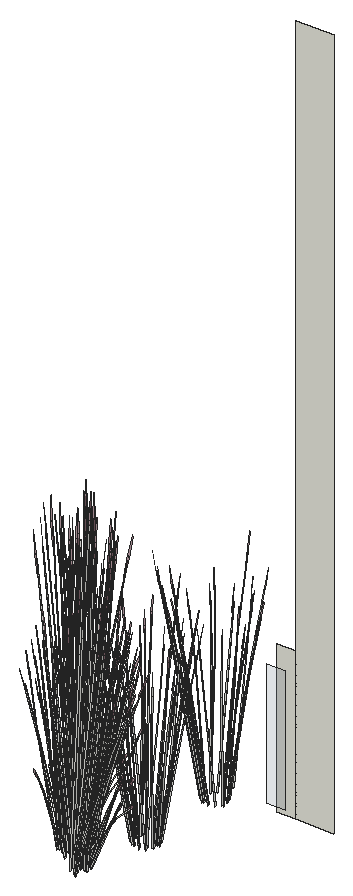
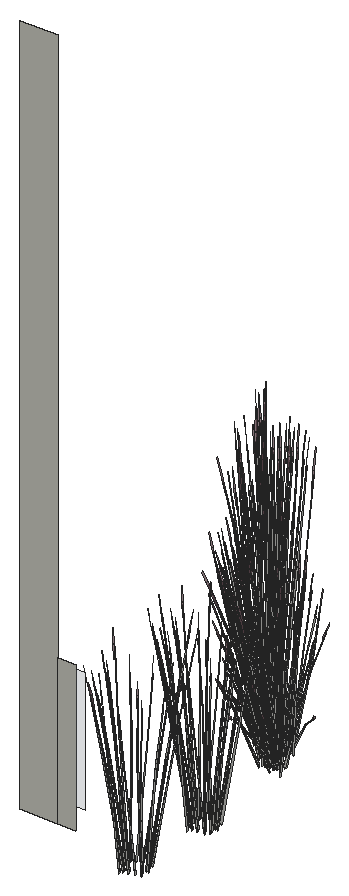
# SketchUp Ruby script. Lengths in inches.
U = 1.inch
M = Sketchup.active_model
def pt(a) = Geom::Point3d.new(a.map { |v| v * U })
def face(e, loops, mat)
  f = e.add_face(loops[0].map { |a| pt(a) })
  loops[1..].each { |l| e.add_face(l.map { |a| pt(a) }).erase! }
  f.material = f.back_material = mat if mat
  f
end
# faces: each face lists its corners as indices into pts; further lists are holes
def faces(e, pts, list, mat = nil) = list.each { |f| face(e, (f[0].is_a?(Array) ? f : [f]).map { |l| l.map { |i| pts[i] } }, mat) }
# xy, xz, yz: faces in a plane at the given z, y or x. An outline is a flat list of corners, or four numbers for a rectangle; further outlines are holes
def ring(l) = l.size == 4 ? [[l[0], l[1]], [l[2], l[1]], [l[2], l[3]], [l[0], l[3]]] : l.each_slice(2).to_a
def flat(e, list, mat, &to3) = list.each { |f| face(e, (f[0].is_a?(Array) ? f : [f]).map { |l| ring(l).map { |u, v| to3.(u, v) } }, mat) }
def xy(e, z, list, mat = nil) = flat(e, list, mat) { |x, y| [x, y, z] }
def xz(e, y, list, mat = nil) = flat(e, list, mat) { |x, z| [x, y, z] }
def yz(e, x, list, mat = nil) = flat(e, list, mat) { |y, z| [x, y, z] }
def lines(e, pts, list) = list.each { |a, b| e.add_line(pt(pts[a]), pt(pts[b])) }
# prism: a flat outline (further loops are holes) pulled along v
def prism(e, loops, v, mat = nil)
  f = face(e, loops, mat); d = Geom::Vector3d.new(v.map { |x| x * U })
  f.pushpull(f.normal.samedirection?(d) ? d.length : -d.length)
end
def box(e, o, s, mat = nil) = prism(e, [[o, [o[0] + s[0], o[1], o[2]], [o[0] + s[0], o[1] + s[1], o[2]], [o[0], o[1] + s[1], o[2]]]], [0, 0, s[2]], mat)
def at(x, y, z, deg = 0) = Geom::Transformation.translation(pt([x, y, z])) * Geom::Transformation.rotation(ORIGIN, Z_AXIS, deg.degrees)
def axes(o, x, y, z) = Geom::Transformation.new([*x, 0, *y, 0, *z, 0, *pt(o).to_a, 1])
def part(name) = M.definitions.add(name)
# library, detail: a bought-in or finely detailed component or shape, given as its bounding box
def library(name, o, s) = part(name).tap { |d| box(d.entities, o, s) }
def detail(e, o, s) = box(e.add_group.entities, o, s)
def put(e, d, t, mat = nil) = e.add_instance(d, t).tap { |i| i.material = mat if mat }
def group(e, t, mat = nil) = e.add_group.tap { |g| g.transformation = t; g.material = mat if mat }.entities
root = M.entities
M.materials.add("D01_Frost_White").color = [238, 238, 227]
M.materials.add("Glass_Basic_01").color = [161, 173, 186]
M.materials["Glass_Basic_01"].alpha = 0.25
M.materials.add("LightPink_Translucent").color = [144, 107, 117]
M.materials["LightPink_Translucent"].alpha = 0.75
c1 = part("blade")
p = [[2.15,0.21,22],[0,0.17,0],[0.09,0.45,0],[2.18,0.31,22],[2.29,0.31,22],[0.38,0.45,0],
  [2.48,0.24,33],[2.49,0.24,33],[2.48,0.22,33]]
faces(c1.entities,p,[[0,1,2,3],[4,5,2,3],[6,3,4,7],[8,0,3,6]])
c2 = part("seeds")
p = [[0.3,-0.1,1.38],[-0.01,-0.03,1.59],[-0.01,-0.03,0.03],[0.14,-0.07,-0.07],[0.29,-0.03,3],[0.15,0.01,3.11]]
faces(c2.entities,p,[[0,1,2,3],[1,0,4,5]],"LightPink_Translucent")
c3 = part("blade with seeds")
put(c3.entities,c1,at(0,0,0))
put(c3.entities,c2,axes([2.4,0.25,30.99],[1.5799,-0.05474,1.17369],[-0.12525,1.92788,0.29478],[-0.07173,-0.02425,1.56792]))
xz(root,674,[[427,158,430,178]],"Glass_Basic_01")
xz(root,676,[[427,156,430,180],[430,156,436,270]],"D01_Frost_White")
put(root,c3,axes([416.55,648.88,157.27],[0.44036,-0.12519,0.14904],[0.10874,0.46588,0.29641],[-0.03927,-0.06788,1.35512]))
put(root,c3,axes([417.46,647.12,157.43],[0.41376,-0.31314,-0.2458],[0.27514,0.44246,-0.42242],[0.10209,0.04493,1.34921]))
put(root,c3,axes([419.1,647.95,159],[0.34057,0.13158,-0.29918],[-0.09933,0.38387,0.38624],[0.13712,-0.0352,0.73904]))
put(root,c3,axes([415.96,649.08,156.88],[-0.38354,-0.23583,-0.41945],[0.22925,-0.42288,0],[-0.08735,-0.05371,1.33059]))
put(root,c3,axes([418.5,646.29,156.88],[0.38354,0.23583,-0.41945],[-0.22925,0.42288,0],[0.08735,0.05371,1.33059]))
put(root,c3,axes([415.1,647.34,159],[-0.34057,-0.13158,-0.29918],[0.09933,-0.38387,0.38624],[-0.13712,0.0352,0.73904]))
put(root,c3,axes([417.78,647.63,157.04],[0.45849,0,0],[0,0.4883,0],[0,0,1.50718]))
put(root,c3,axes([417,648.25,157.43],[-0.41376,0.31314,-0.2458],[-0.27514,-0.44246,-0.42242],[-0.10209,-0.04493,1.34921]))
put(root,c3,axes([417.91,646.49,157.27],[-0.44036,0.12519,0.14904],[-0.10874,-0.46588,0.29641],[0.03927,0.06788,1.35512]))
put(root,c3,axes([418.18,647.47,158.45],[-0.16998,0.01068,1.44779],[0.11276,-0.46299,0.11706],[0.24224,0.02864,0.61892]))
put(root,c3,axes([418.4,646.46,156.89],[0.09626,0.41098,-0.2617],[-0.38233,0.1167,0.2617],[0.07708,0.04739,1.17405]))
put(root,c3,axes([419.05,648.11,159.17],[0.15051,0.3216,0.05432],[-0.27447,0.15741,0.42765],[0.12099,-0.03106,0.65209]))
put(root,c3,axes([417.63,647.39,157.19],[-0.51796,-0.09937,0.41563],[0.10541,-0.56124,0.1631],[0.07569,0.05419,1.44303]))
put(root,c3,axes([419.03,647.99,159.18],[-0.11578,0.43006,0.40553],[-0.38064,-0.14706,0.33437],[0.14969,-0.02584,0.83914]))
put(root,c3,axes([417.21,648.77,157.04],[-0.13371,-0.40664,0],[0.38182,-0.1424,0],[0,0,1.30413]))
put(root,c3,axes([416.96,648.39,157.39],[-0.07906,0.42093,0.12232],[-0.38625,-0.07307,-0.3493],[-0.07029,-0.04322,1.07074]))
put(root,c3,axes([415.46,647.29,159.45],[0.34057,0.13158,0.29918],[-0.09933,0.38387,-0.38624],[-0.13712,0.0352,0.73904]))
put(root,c3,axes([417.71,648.71,157.02],[0.43024,-0.16003,-0.16218],[0.15118,0.46099,0.00007],[0.04749,-0.01769,1.46908]))
put(root,c3,axes([417.86,648.91,157.27],[0.11838,-0.46875,0.14904],[0.43321,0.13265,0.29641],[-0.07483,0.00228,1.35512]))
put(root,c3,axes([417.77,647.84,157.05],[0.28606,0.30466,0],[-0.28606,0.30466,0],[0,0,1.42996]))
put(root,c3,axes([416.14,647.27,158],[0.11649,-0.06823,1.49584],[0.04017,0.47639,0.11706],[-0.25231,0.06321,0.53462]))
put(root,c3,axes([418.54,647.71,157.27],[-0.32198,-0.34356,0.14904],[0.32447,-0.33323,0.29641],[-0.03556,0.07016,1.35512]))
put(root,c3,axes([417.94,647.19,156.92],[0.42629,0.07733,-0.52676],[-0.08996,0.47699,-0.13825],[0.12722,0.0578,1.16273]))
put(root,c3,axes([419.83,648.02,157.51],[-0.2532,0.07787,0.97034],[0.11918,-0.32181,0.71294],[0.13432,0.02202,0.21373]))
put(root,c3,axes([417.12,648.95,157.03],[-0.41314,-0.21175,0],[0.19883,-0.43999,0],[0,0,1.37455]))
put(root,c3,axes([417.46,648.39,157.26],[-0.40016,-0.37963,-0.21282],[0.33672,-0.42629,0.46574],[-0.10776,0.04441,1.42109]))
put(root,c3,axes([416.41,649.12,157.27],[0.38354,0.23583,0.41945],[-0.22925,0.42288,0],[-0.08735,-0.05371,1.33059]))
put(root,c3,axes([417.76,647.49,157.48],[0.19883,-0.425,0.37796],[0.41314,0.20454,-0.1819],[0,0.09797,1.2135]))
put(root,c3,axes([419.71,649.39,159.16],[-0.03706,-0.04129,1.49853],[0.08106,-0.44261,-0.1416],[0.14596,-0.02828,0.26519]))
put(root,c3,axes([414.89,647.59,159.16],[-0.06692,0.06124,1.47793],[0.00569,0.44742,-0.23373],[-0.15339,0.05818,0.11853]))
put(root,c3,axes([417.68,647.73,157.12],[0,0.54548,-0.04762],[-0.51243,0,0],[0,0.01714,1.5153]))
put(root,c3,axes([415.34,647.53,159.13],[-0.11102,0.42903,-0.43168],[-0.38064,-0.14706,-0.33437],[-0.15325,0.03934,0.82598]))
put(root,c3,axes([415.32,647.16,159.43],[0.20619,0.42709,-0.10273],[-0.36595,0.20988,-0.57019],[-0.15422,0.05635,0.8664]))
put(root,c3,axes([417.72,647.34,157.05],[0.24618,0.39589,-0.37796],[-0.37289,0.27878,0.1819],[0.07967,0.04899,1.2135]))
put(root,c3,axes([419.39,649.02,158.5],[-0.07843,-0.39649,-0.0295],[0.37072,-0.09115,-0.13375],[0.07742,0.02514,0.44114]))
put(root,c3,axes([416.1875,649.37,157.18],[-0.25622,0.47263,0],[-0.42866,-0.26357,-0.43598],[-0.09763,-0.06003,1.38303]))
put(root,c3,axes([418.43,649,159.43],[0.02194,-0.47967,-0.10273],[0.41546,0.01311,-0.57019],[0.16001,0.03332,0.8664]))
put(root,c3,axes([418.8,647.72,157.27],[0,-0.47166,0.41945],[0.45849,0,0],[0,0.10742,1.33059]))
put(root,c3,axes([417.66,648.08,157.48],[0.44501,-0.02912,0.37796],[0.04024,0.48332,-0.1819],[-0.07967,0.04899,1.2135]))
put(root,c3,axes([417.93,647.58,157.39],[0.38182,-0.13755,0.12232],[0.13371,0.39278,-0.3493],[0,0.08644,1.07074]))
put(root,c3,axes([418.36,648.82,159.45],[-0.23317,-0.29531,0.29918],[0.26625,-0.27955,-0.38624],[0.13527,0.04253,0.73904]))
put(root,c3,axes([417.26,648.3125,157.05],[-0.44501,0.02912,-0.37796],[-0.04024,-0.48332,0.1819],[-0.07967,0.04899,1.2135]))
put(root,c3,axes([419.35,648.54,157.37],[-0.0987,-0.116,1.20808],[0.12841,-0.38374,-0.25981],[0.19968,0.05198,0.51652]))
put(root,c3,axes([417.59,648.96,157.04],[0.41314,0.21175,0],[-0.19883,0.43999,0],[0,0,1.47801]))
put(root,c3,axes([418.79,648.72,159.16],[0.08791,-0.00798,1.47793],[0.24113,-0.36643,-0.23373],[0.15637,0.04837,0.11853]))
put(root,c3,axes([417.75,649.43,157.03],[-0.25302,-0.47428,-0.04344],[0.42866,-0.26357,0.43598],[-0.10563,0.04516,1.38235]))
put(root,c3,axes([417.66,648.28,157.39],[0.30276,0.28338,0.12232],[-0.25254,0.31972,-0.3493],[-0.07029,0.04322,1.07074]))
put(root,c3,axes([415.27,648.36,159.18],[-0.10163,-0.43409,0.40553],[0.39868,-0.07534,0.33437],[-0.1175,0.10209,0.83914]))
put(root,c3,axes([415.19,648.28,159.17],[-0.28133,-0.19836,0.05432],[0.16379,-0.28248,0.42765],[-0.0902,0.09132,0.65209]))
put(root,c3,axes([415.32,647.75,158.45],[0.14219,-0.09977,1.44779],[0.11971,0.461,0.11706],[-0.22323,0.10419,0.61892]))
put(root,c3,axes([418.45,648.77,159.39],[0.40965,0.01136,-0.60019],[-0.02751,0.47821,0.07243],[0.17355,0.05047,0.84903]))
put(root,c3,axes([417.99,649.16,157.27],[0.38354,-0.23583,0.41945],[0.22925,0.42288,0],[-0.08735,0.05371,1.33059]))
put(root,c3,axes([417.44,648.79,157.11],[0.17817,0.54185,-0.05079],[-0.50909,0.18987,0],[0.00622,0.01892,1.45452]))
put(root,c3,axes([417.64,649.37,156.89],[-0.38233,-0.1167,-0.2617],[0.09626,-0.41098,0.2617],[-0.07708,0.04739,1.17405]))
put(root,c3,axes([414.88,648.54,157.37],[0.14242,0.03872,1.20808],[0.09179,0.39548,-0.25981],[-0.19345,0.07403,0.51652]))
put(root,c3,axes([415.52,648.21,159.45],[0.35672,-0.06741,0.29918],[0.09419,0.38534,-0.38624],[-0.10222,0.1035,0.73904]))
put(root,c3,axes([419.12,647.8,157.1875],[0.51243,0,0],[0,0.52715,-0.43598],[0,0.12006,1.38303]))
put(root,c3,axes([414.14,648.04,159.16],[0.0523,0.01265,1.49853],[0.16179,0.41674,-0.1416],[-0.10706,0.10938,0.26519]))
put(root,c3,axes([418.91,648.07,157.04],[-0.51218,-0.00377,-0.04204],[0,-0.52715,0.42192],[-0.0161,0.12,1.33776]))
put(root,c3,axes([417.8,647.62,157.43],[0.46151,0.22505,-0.2458],[-0.22222,0.475,-0.42242],[0.0145,0.11662,1.34921]))
put(root,c3,axes([414.58,649.37,157.51],[0.17079,-0.21377,0.97034],[0.06739,0.33841,0.71294],[-0.12342,0.0606,0.21373]))
put(root,c3,axes([418.69,648.97,159],[0.23317,0.29531,-0.29918],[-0.26625,0.27955,0.38624],[0.13527,0.04253,0.73904]))
put(root,c3,axes([418.8,648.15,156.89],[-0.28606,0.29428,-0.2617],[-0.28606,-0.29428,0.2617],[0,0.09479,1.17405]))
put(root,c3,axes([417.57,648.18,157.43],[0.04775,0.53819,-0.2458],[-0.49736,0.03254,-0.42242],[-0.08758,0.07169,1.34921]))
put(root,c3,axes([418.57,649.08,159.17],[-0.02064,0.35866,0.05432],[-0.3116,-0.00983,0.42765],[0.11936,0.03753,0.65209]))
put(root,c3,axes([417.75,647.97,157.05],[-0.19883,0.425,-0.37796],[-0.41314,-0.20454,0.1819],[0,0.09797,1.2135]))
put(root,c3,axes([415.23,648.44,159],[-0.35672,0.06741,-0.29918],[-0.09419,-0.38534,0.38624],[-0.10222,0.1035,0.73904]))
put(root,c3,axes([418.6,648.97,159.18],[-0.30217,0.31079,0.40553],[-0.2606,-0.33005,0.33437],[0.14177,0.05733,0.83914]))
put(root,c3,axes([414.71,649.31,159.95],[0.36162,0.1259,-0.05481],[-0.11124,0.3875,-0.2485],[-0.05915,0.05883,0.81966]))
put(root,c3,axes([417.27,648.59,156.92],[-0.27603,0.35451,-0.52676],[-0.34289,-0.32147,-0.13825],[-0.11061,0.08844,1.16273]))
put(root,c3,axes([417.64,649.33,159.45],[-0.06329,-0.37991,0.29918],[0.36182,-0.10032,-0.38624],[0.09718,0.10887,0.73904]))
put(root,c3,axes([417.76,649.1875,157.15],[0.51304,0.1533,0.25983],[-0.12835,0.54797,-0.30828],[-0.08491,0.06858,1.39295]))
put(root,c3,axes([417.73,649.56,156.88],[-0.38354,0.23583,-0.41945],[-0.22925,-0.42288,0],[-0.08735,0.05371,1.33059]))
put(root,c3,axes([419,648.16,156.88],[0,0.47166,-0.41945],[-0.45849,0,0],[0,0.10742,1.33059]))
put(root,c3,axes([417.86,648.21,158.45],[-0.15222,-0.08126,1.44779],[0.31502,-0.34091,0.11706],[0.19634,0.15379,0.61892]))
put(root,c3,axes([417.88,647.14,158.96],[-0.35411,-0.24507,1.16821],[0.37391,-0.38156,0.50405],[0.11425,0.22994,1.12919]))
put(root,c3,axes([415.33,648.18,159.43],[0.37908,0.26007,-0.10273],[-0.21839,0.37663,-0.57019],[-0.1071,0.13092,0.8664]))
put(root,c3,axes([418.42,649.14,157.51],[-0.23074,-0.13562,0.97034],[0.29794,-0.1378,0.71294],[0.08036,0.11673,0.21373]))
put(root,c3,axes([417.61,649.53,159.43],[0.2442,-0.40372,-0.10273],[0.35364,0.23259,-0.57019],[0.12293,0.11406,0.8664]))
put(root,c3,axes([415.84,648.0625,158.45],[0.10236,-0.14492,1.44779],[0.25844,0.39118,0.11706],[-0.17726,0.17814,0.61892]))
put(root,c3,axes([415.52,648.49,159.13],[0.10528,0.43067,-0.43168],[-0.39868,0.07534,-0.33437],[-0.11425,0.11568,0.82598]))
put(root,c3,axes([416,648.98,159.45],[0.27728,-0.24833,0.29918],[0.26248,0.28355,-0.38624],[-0.03994,0.14407,0.73904]))
put(root,c3,axes([418.08,649.48,157.18],[0.25622,0.47263,0],[-0.42866,0.26357,-0.43598],[-0.09763,0.06003,1.38303]))
put(root,c3,axes([417.29,649.86,159.16],[0.00121,-0.0571,1.49853],[0.35119,-0.25193,-0.1416],[0.12199,0.08992,0.26519]))
put(root,c3,axes([418.48,649.64,156.44],[0.02986,-0.06809,1.48974],[0.37589,-0.20055,-0.22758],[0.11396,0.1038,0.25375]))
put(root,c3,axes([417.86,647.61,157.58],[-0.01119,-0.44408,1.19347],[0.50665,0.11511,0.50532],[-0.11983,0.243,1.12654]))
put(root,c3,axes([417.99,648.1,156.95],[0.15027,0.43184,-0.5847],[-0.43285,0.15553,-0.15346],[0.01661,0.14623,1.29063]))
put(root,c3,axes([415.75,649.21,159.17],[-0.33677,-0.02198,0.05432],[0.00923,-0.33185,0.42765],[-0.03524,0.12712,0.65209]))
put(root,c3,axes([415.03,649.59,156.44],[0.05497,0.04712,1.48974],[0.09321,0.43661,-0.22758],[-0.12183,0.0931,0.25375]))
put(root,c3,axes([415.85,649.24,159.18],[-0.29182,-0.32181,0.40553],[0.3099,-0.27755,0.33437],[-0.05383,0.15098,0.83914]))
put(root,c3,axes([417.9,649.33,159.13],[0.40438,-0.11212,-0.43168],[0.07074,0.4246,-0.33437],[0.10862,0.12168,0.82598]))
put(root,c3,axes([416.78,649.39,159.45],[0.12355,-0.36271,0.29918],[0.36044,0.10579,-0.38624],[0.03305,0.14603,0.73904]))
put(root,c3,axes([418.46,649.76,157.43],[-0.26279,-0.01479,0.88755],[0.17355,-0.31417,0.49003],[0.10382,0.11162,0.6962]))
put(root,c3,axes([417.7,649.67,159.17],[-0.18625,0.29962,0.05432],[-0.26523,-0.17444,0.42765],[0.08575,0.09606,0.65209]))
put(root,c3,axes([417.26,650.68,159.95],[0.28319,-0.27058,-0.05481],[0.25948,0.29635,-0.2485],[0.01827,0.08397,0.81966]))
put(root,c3,axes([417.78,649.59,159.18],[-0.4076,0.10824,0.40553],[-0.07074,-0.4246,0.33437],[0.09586,0.12514,0.83914]))
put(root,c3,axes([415.77,648.42,158.45],[0.0763,-0.16212,1.44779],[0.3201,0.3355,0.11706],[-0.1444,0.2091,0.61892]))
put(root,c3,axes([417.6,649,157.37],[0.00723,-0.15635,1.20808],[0.34559,-0.17464,-0.25981],[0.10668,0.18713,0.51652]))
put(root,c3,axes([416.66,649.72,159.17],[-0.30197,0.1603,0.05432],[-0.1478,-0.29231,0.42765],[0.02916,0.12885,0.65209]))
put(root,c3,axes([415.85,649.33,159],[-0.27728,0.24833,-0.29918],[-0.26248,-0.28355,0.38624],[-0.03994,0.14407,0.73904]))
put(root,c3,axes([414.9,649.26,159.16],[-0.01019,0.09334,1.47793],[0.28908,0.3247,-0.23373],[-0.07568,0.15355,0.11853]))
put(root,c3,axes([415.82,649.05,159.74],[0.45039,0.02337,-0.11403],[-0.01231,0.44247,-0.63292],[-0.03129,0.17041,0.9617]))
put(root,c3,axes([416.66,649.54,159.43],[0.40102,-0.2196,-0.10273],[0.19707,0.38974,-0.57019],[0.05291,0.16424,0.8664]))
put(root,c3,axes([416.77,649.6875,159.46],[-0.4038,-0.12331,0.45013],[0.13808,-0.40538,0.37115],[0.02427,0.15942,0.93144]))
put(root,c3,axes([416.03,650.3,157.51],[-0.01061,-0.28045,0.97034],[0.26501,0.20003,0.71294],[-0.05212,0.13367,0.21373]))
put(root,c3,axes([416.73,649.63,156.44],[0.06632,-0.02567,1.48974],[0.39894,0.14126,-0.22758],[0.01167,0.15921,0.25375]))
put(root,c3,axes([416.13,649.22,159.41],[0.29336,0.31691,-0.47917],[-0.3099,0.27755,-0.37115],[-0.04464,0.16102,0.91684]))
put(root,c3,axes([415.8125,649.69,157.5625],[0.37228,-0.08352,0.05498],[0.08559,0.3365,-0.7291],[-0.0236,0.17034,0.65354]))
put(root,c3,axes([417,649.52,159.13],[0.40284,0.11824,-0.43168],[-0.13808,0.40538,-0.33437],[0.03694,0.16321,0.82598]))
put(root,c3,axes([417.23,648.6875,158.45],[-0.09368,-0.15143,1.44779],[0.43286,-0.12749,0.11706],[0.09783,0.23774,0.61892]))
put(root,c3,axes([416.82,649.77,159],[-0.12355,0.36271,-0.29918],[-0.36044,-0.10579,0.38624],[0.03305,0.14603,0.73904]))
put(root,c3,axes([416.04,649.07,159.6875],[-0.01066,0.43628,-0.66621],[-0.44902,-0.0293,0.0804],[-0.04739,0.18483,0.94242]))
put(root,c3,axes([414.87,650.22,159.16],[0.04649,-0.02848,1.49853],[0.38427,0.18941,-0.1416],[-0.00903,0.15771,0.26519]))
put(root,c3,axes([416.46,648.76,158.45],[-0.01003,-0.18103,1.44779],[0.43473,0.12009,0.11706],[-0.02689,0.25798,0.61892]))
put(root,c3,axes([416.85,649.45,159.39],[0.19559,0.38351,-0.60019],[-0.40262,0.21373,0.07243],[0.04574,0.1853,0.84903]))
put(root,c3,axes([415.72,650.05,157.37],[0.12932,-0.07441,1.20808],[0.31929,0.22435,-0.25981],[-0.09503,0.19413,0.51652]))
put(root,c3,axes([416.5625,650.42,159.16],[0.05195,0.07595,1.47793],[0.41921,0.02984,-0.23373],[0.04216,0.1675,0.11853]))
put(root,c3,axes([415.89,649.6875,158.02],[0.009,-0.24349,1.30391],[0.40497,0.12861,0.18019],[-0.03509,0.2595,0.61571]))
put(root,c3,axes([416.4,660.26,154.3],[0.45651,-0.12123,0.45419],[0.07923,0.47555,0.3745],[-0.10736,-0.14016,0.93983]))
put(root,c3,axes([417.43,660.35,154],[0.4038,0.12331,0.40553],[-0.13808,0.40538,0.33437],[-0.02427,-0.15942,0.83914]))
put(root,c3,axes([417.43,660.65,154.27],[-0.12355,0.36271,0.29918],[-0.36044,-0.10579,-0.38624],[-0.03305,-0.14603,0.73904]))
put(root,c3,axes([418.35,660.8,154],[0.29182,0.32181,0.40553],[-0.3099,0.27755,0.33437],[0.05383,-0.15098,0.83914]))
put(root,c3,axes([418.21,661.05,154.27],[-0.27728,0.24833,0.29918],[-0.26248,-0.28355,-0.38624],[0.03994,-0.14407,0.73904]))
put(root,c3,axes([416.56,660.71,154.27],[0.06329,0.37991,0.29918],[-0.36182,0.10032,-0.38624],[-0.09718,-0.10887,0.73904]))
put(root,c3,axes([415.48,660.95,154.3],[0.33843,-0.34808,0.45419],[0.29188,0.36965,0.3745],[-0.15878,-0.06421,0.93983]))
put(root,c3,axes([418.6875,661.82,154.27],[-0.35672,0.06741,0.29918],[-0.09419,-0.38534,-0.38624],[0.10222,-0.1035,0.73904]))
put(root,c3,axes([418.93,661.68,154],[0.10163,0.43409,0.40553],[-0.39868,0.07534,0.33437],[0.1175,-0.10209,0.83914]))
put(root,c3,axes([415.84,661.22,154.27],[0.23317,0.29531,0.29918],[-0.26625,0.27955,-0.38624],[-0.13527,-0.04253,0.73904]))
put(root,c3,axes([418.75,662.74,154.27],[-0.34057,-0.13158,0.29918],[0.09933,-0.38387,-0.38624],[0.13712,-0.0352,0.73904]))
put(root,c3,axes([415.18,662.04,154],[0.11578,-0.43006,0.40553],[0.38064,0.14706,0.33437],[-0.14969,0.02584,0.83914]))
put(root,c3,axes([419.03,662.75,154],[-0.11578,0.43006,0.40553],[-0.38064,-0.14706,0.33437],[0.14969,-0.02584,0.83914]))
put(root,c3,axes([415.46,662.05,154.27],[0.34057,0.13158,0.29918],[-0.09933,0.38387,-0.38624],[-0.13712,0.0352,0.73904]))
put(root,c3,axes([418.36,663.57,154.27],[-0.23317,-0.29531,0.29918],[0.26625,-0.27955,-0.38624],[0.13527,0.04253,0.73904]))
put(root,c3,axes([415.27,663.11,154],[-0.10163,-0.43409,0.40553],[0.39868,-0.07534,0.33437],[-0.1175,0.10209,0.83914]))
put(root,c3,axes([415.52,662.97,154.27],[0.35672,-0.06741,0.29918],[0.09419,0.38534,-0.38624],[-0.10222,0.1035,0.73904]))
put(root,c3,axes([418.6,663.72,154],[-0.30217,0.31079,0.40553],[-0.2606,-0.33005,0.33437],[0.14177,0.05733,0.83914]))
put(root,c3,axes([414.71,664.0625,154.77],[0.36162,0.1259,-0.05481],[-0.11124,0.3875,-0.2485],[-0.05915,0.05883,0.81966]))
put(root,c3,axes([417.64,664.08,154.27],[-0.06329,-0.37991,0.29918],[0.36182,-0.10032,-0.38624],[0.09718,0.10887,0.73904]))
put(root,c3,axes([416,663.74,154.27],[0.27728,-0.24833,0.29918],[0.26248,0.28355,-0.38624],[-0.03994,0.14407,0.73904]))
put(root,c3,axes([415.85,663.99,154],[-0.29182,-0.32181,0.40553],[0.3099,-0.27755,0.33437],[-0.05383,0.15098,0.83914]))
put(root,c3,axes([416.78,664.14,154.27],[0.12355,-0.36271,0.29918],[0.36044,0.10579,-0.38624],[0.03305,0.14603,0.73904]))
put(root,c3,axes([417.26,665.4375,154.77],[0.28319,-0.27058,-0.05481],[0.25948,0.29635,-0.2485],[0.01827,0.08397,0.81966]))
put(root,c3,axes([417.78,664.34,154],[-0.4076,0.10824,0.40553],[-0.07074,-0.4246,0.33437],[0.09586,0.12514,0.83914]))
put(root,c3,axes([416.77,664.44,154.28],[-0.4038,-0.12331,0.45013],[0.13808,-0.40538,0.37115],[0.02427,0.15942,0.93144]))
put(root,c3,axes([416.4,674.14,154.3],[0.45651,-0.12123,0.45419],[0.07923,0.47555,0.3745],[-0.10736,-0.14016,0.93983]))
put(root,c3,axes([417.43,674.52,154.27],[-0.12355,0.36271,0.29918],[-0.36044,-0.10579,-0.38624],[-0.03305,-0.14603,0.73904]))
put(root,c3,axes([418.21,674.93,154.27],[-0.27728,0.24833,0.29918],[-0.26248,-0.28355,-0.38624],[0.03994,-0.14407,0.73904]))
put(root,c3,axes([416.56,674.58,154.27],[0.06329,0.37991,0.29918],[-0.36182,0.10032,-0.38624],[-0.09718,-0.10887,0.73904]))
put(root,c3,axes([415.48,674.83,154.3],[0.33843,-0.34808,0.45419],[0.29188,0.36965,0.3745],[-0.15878,-0.06421,0.93983]))
put(root,c3,axes([418.6875,675.7,154.27],[-0.35672,0.06741,0.29918],[-0.09419,-0.38534,-0.38624],[0.10222,-0.1035,0.73904]))
put(root,c3,axes([418.93,675.55,154],[0.10163,0.43409,0.40553],[-0.39868,0.07534,0.33437],[0.1175,-0.10209,0.83914]))
put(root,c3,axes([415.84,675.1,154.27],[0.23317,0.29531,0.29918],[-0.26625,0.27955,-0.38624],[-0.13527,-0.04253,0.73904]))
put(root,c3,axes([418.75,676.62,154.27],[-0.34057,-0.13158,0.29918],[0.09933,-0.38387,-0.38624],[0.13712,-0.0352,0.73904]))
put(root,c3,axes([415.18,675.92,154],[0.11578,-0.43006,0.40553],[0.38064,0.14706,0.33437],[-0.14969,0.02584,0.83914]))
put(root,c3,axes([415.46,675.92,154.27],[0.34057,0.13158,0.29918],[-0.09933,0.38387,-0.38624],[-0.13712,0.0352,0.73904]))
put(root,c3,axes([418.36,677.45,154.27],[-0.23317,-0.29531,0.29918],[0.26625,-0.27955,-0.38624],[0.13527,0.04253,0.73904]))
put(root,c3,axes([415.52,676.84,154.27],[0.35672,-0.06741,0.29918],[0.09419,0.38534,-0.38624],[-0.10222,0.1035,0.73904]))
put(root,c3,axes([414.71,677.9375,154.77],[0.36162,0.1259,-0.05481],[-0.11124,0.3875,-0.2485],[-0.05915,0.05883,0.81966]))
put(root,c3,axes([417.64,677.96,154.27],[-0.06329,-0.37991,0.29918],[0.36182,-0.10032,-0.38624],[0.09718,0.10887,0.73904]))
put(root,c3,axes([416,677.61,154.27],[0.27728,-0.24833,0.29918],[0.26248,0.28355,-0.38624],[-0.03994,0.14407,0.73904]))
put(root,c3,axes([416.78,678.02,154.27],[0.12355,-0.36271,0.29918],[0.36044,0.10579,-0.38624],[0.03305,0.14603,0.73904]))
put(root,c3,axes([417.26,679.31,154.77],[0.28319,-0.27058,-0.05481],[0.25948,0.29635,-0.2485],[0.01827,0.08397,0.81966]))
put(root,c3,axes([417.78,678.22,154],[-0.4076,0.10824,0.40553],[-0.07074,-0.4246,0.33437],[0.09586,0.12514,0.83914]))
put(root,c3,axes([416.77,678.32,154.28],[-0.4038,-0.12331,0.45013],[0.13808,-0.40538,0.37115],[0.02427,0.15942,0.93144]))
